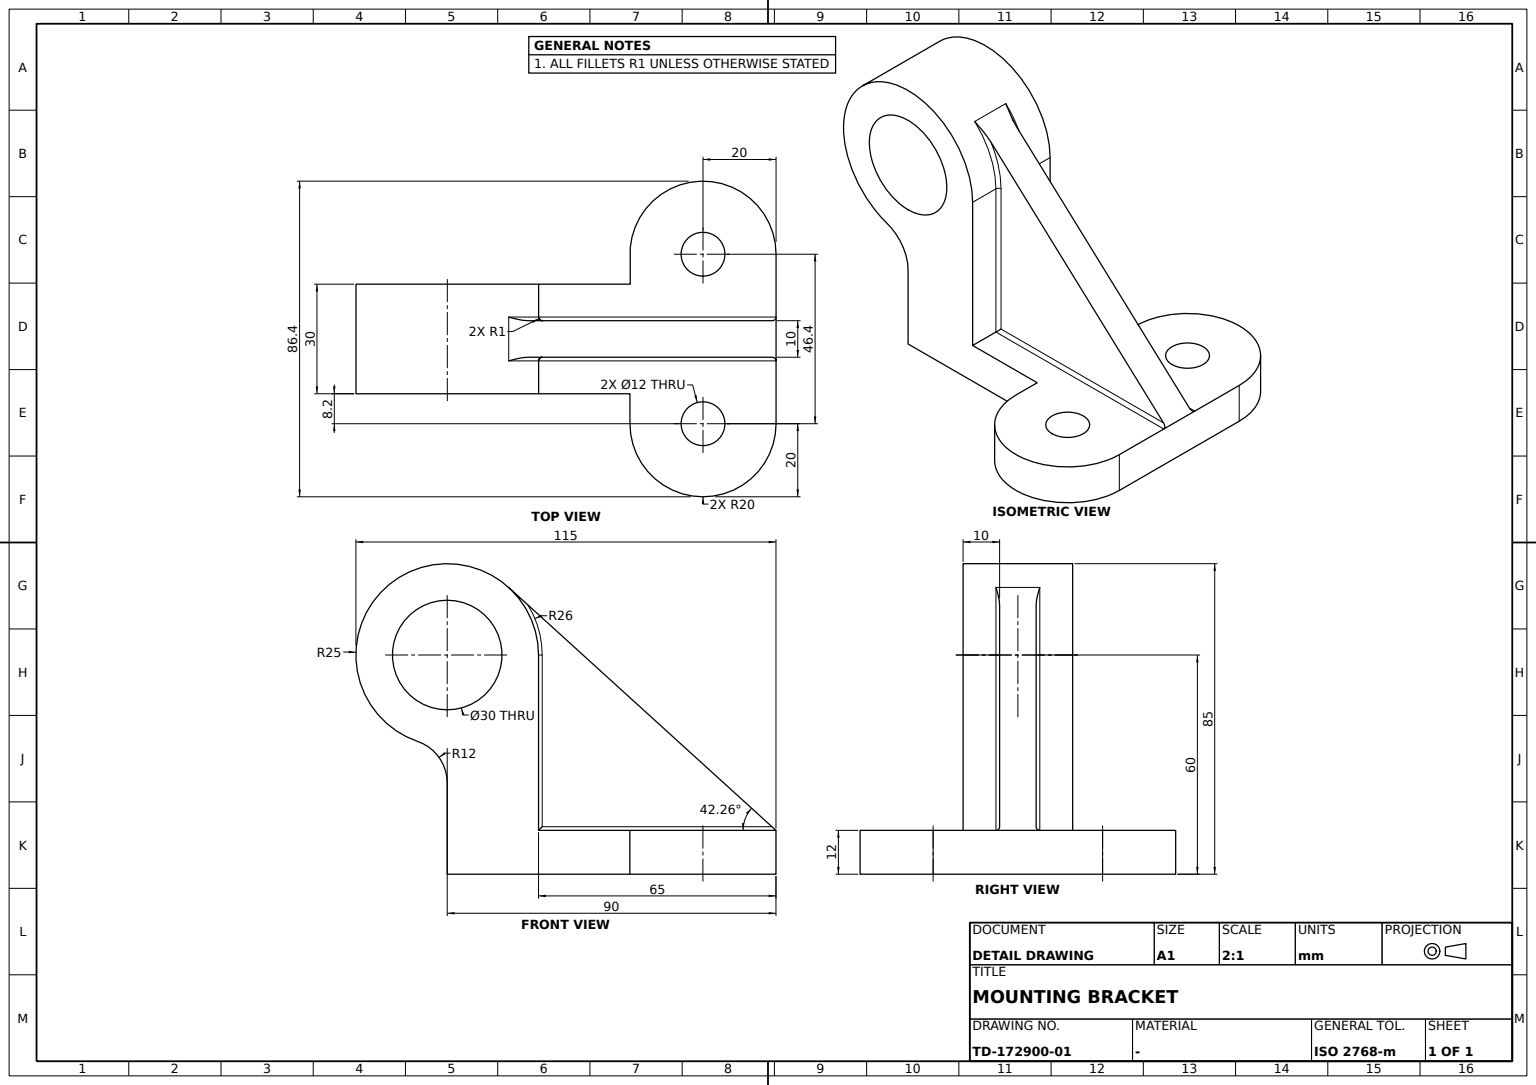
ISO-10303-21;
HEADER;
FILE_DESCRIPTION((''),'2;1');
FILE_NAME('','',(''),(''),'','','');
FILE_SCHEMA(('AUTOMOTIVE_DESIGN'));
ENDSEC;
DATA;
#1=APPLICATION_CONTEXT('');
#2=PRODUCT_CONTEXT('',#1,'mechanical');
#3=PRODUCT('','','',(#2));
#4=PRODUCT_DEFINITION_FORMATION('','',#3);
#5=PRODUCT_DEFINITION_CONTEXT('',#1,'design');
#6=PRODUCT_DEFINITION('','',#4,#5);
#7=PRODUCT_DEFINITION_SHAPE('','',#6);
#8=(LENGTH_UNIT()NAMED_UNIT(*)SI_UNIT(.MILLI.,.METRE.));
#9=(NAMED_UNIT(*)PLANE_ANGLE_UNIT()SI_UNIT($,.RADIAN.));
#10=(NAMED_UNIT(*)SI_UNIT($,.STERADIAN.)SOLID_ANGLE_UNIT());
#11=UNCERTAINTY_MEASURE_WITH_UNIT(LENGTH_MEASURE(0.005),#8,'distance_accuracy_value','');
#12=(GEOMETRIC_REPRESENTATION_CONTEXT(3)GLOBAL_UNCERTAINTY_ASSIGNED_CONTEXT((#11))GLOBAL_UNIT_ASSIGNED_CONTEXT((#8,#9,#10))REPRESENTATION_CONTEXT('',''));
#13=CARTESIAN_POINT('',(23.199566,90.,-60.));
#14=VERTEX_POINT('',#13);
#15=CARTESIAN_POINT('',(23.199566,90.,-48.));
#16=VERTEX_POINT('',#15);
#17=CARTESIAN_POINT('',(23.199566,90.,-54.));
#18=DIRECTION('',(0.,0.,1.));
#19=VECTOR('',#18,1000.);
#20=LINE('',#17,#19);
#21=EDGE_CURVE('',#14,#16,#20,.T.);
#22=ORIENTED_EDGE('',*,*,#21,.F.);
#23=CARTESIAN_POINT('',(-23.199566,90.,-60.));
#24=VERTEX_POINT('',#23);
#25=CARTESIAN_POINT('',(0.,90.,-60.));
#26=DIRECTION('',(1.,0.,0.));
#27=VECTOR('',#26,1000.);
#28=LINE('',#25,#27);
#29=EDGE_CURVE('',#24,#14,#28,.T.);
#30=ORIENTED_EDGE('',*,*,#29,.F.);
#31=CARTESIAN_POINT('',(-23.199566,90.,-48.));
#32=VERTEX_POINT('',#31);
#33=CARTESIAN_POINT('',(-23.199566,90.,-54.));
#34=LINE('',#33,#19);
#35=EDGE_CURVE('',#24,#32,#34,.T.);
#36=ORIENTED_EDGE('',*,*,#35,.T.);
#37=CARTESIAN_POINT('',(-6.,90.,-48.));
#38=VERTEX_POINT('',#37);
#39=CARTESIAN_POINT('',(0.,90.,-48.));
#40=LINE('',#39,#27);
#41=EDGE_CURVE('',#32,#38,#40,.T.);
#42=ORIENTED_EDGE('',*,*,#41,.T.);
#43=CARTESIAN_POINT('',(6.,90.,-48.));
#44=VERTEX_POINT('',#43);
#45=LINE('',#31,#27);
#46=EDGE_CURVE('',#38,#44,#45,.T.);
#47=ORIENTED_EDGE('',*,*,#46,.T.);
#48=EDGE_CURVE('',#44,#16,#40,.T.);
#49=ORIENTED_EDGE('',*,*,#48,.T.);
#50=EDGE_LOOP('',(#22,#30,#36,#42,#47,#49));
#51=FACE_BOUND('',#50,.T.);
#52=DIRECTION('',(0.,-1.,0.));
#53=AXIS2_PLACEMENT_3D('',#23,#52,#26);
#54=PLANE('',#53);
#55=ADVANCED_FACE('',(#51),#54,.F.);
#56=CARTESIAN_POINT('',(-15.,0.,-15.));
#57=VERTEX_POINT('',#56);
#58=CARTESIAN_POINT('',(-15.,0.,0.));
#59=DIRECTION('',(0.,0.,-1.));
#60=AXIS2_PLACEMENT_3D('',#58,#26,#59);
#61=CIRCLE('',#60,15.);
#62=EDGE_CURVE('',#57,#57,#61,.T.);
#63=ORIENTED_EDGE('',*,*,#62,.F.);
#64=EDGE_LOOP('',(#63));
#65=FACE_BOUND('',#64,.T.);
#66=CARTESIAN_POINT('',(15.,0.,-15.));
#67=VERTEX_POINT('',#66);
#68=CARTESIAN_POINT('',(15.,0.,0.));
#69=AXIS2_PLACEMENT_3D('',#68,#26,#59);
#70=CIRCLE('',#69,15.);
#71=EDGE_CURVE('',#67,#67,#70,.T.);
#72=ORIENTED_EDGE('',*,*,#71,.T.);
#73=EDGE_LOOP('',(#72));
#74=FACE_BOUND('',#73,.T.);
#75=CARTESIAN_POINT('',(0.,0.,0.));
#76=DIRECTION('',(0.,1.,0.));
#77=AXIS2_PLACEMENT_3D('',#75,#26,#76);
#78=CYLINDRICAL_SURFACE('',#77,15.);
#79=ADVANCED_FACE('',(#65,#74),#78,.F.);
#80=CARTESIAN_POINT('',(29.199566,70.,-60.));
#81=VERTEX_POINT('',#80);
#82=CARTESIAN_POINT('',(23.199566,70.,-60.));
#83=AXIS2_PLACEMENT_3D('',#82,#18,#26);
#84=CIRCLE('',#83,6.);
#85=EDGE_CURVE('',#81,#81,#84,.T.);
#86=ORIENTED_EDGE('',*,*,#85,.T.);
#87=EDGE_LOOP('',(#86));
#88=FACE_BOUND('',#87,.T.);
#89=CARTESIAN_POINT('',(23.199566,50.,-60.));
#90=VERTEX_POINT('',#89);
#91=CIRCLE('',#83,20.);
#92=EDGE_CURVE('',#90,#14,#91,.T.);
#93=ORIENTED_EDGE('',*,*,#92,.F.);
#94=CARTESIAN_POINT('',(15.,50.,-60.));
#95=VERTEX_POINT('',#94);
#96=CARTESIAN_POINT('',(0.,50.,-60.));
#97=DIRECTION('',(-1.,0.,0.));
#98=VECTOR('',#97,1000.);
#99=LINE('',#96,#98);
#100=EDGE_CURVE('',#90,#95,#99,.T.);
#101=ORIENTED_EDGE('',*,*,#100,.T.);
#102=CARTESIAN_POINT('',(15.,0.,-60.));
#103=VERTEX_POINT('',#102);
#104=VECTOR('',#52,1000.);
#105=LINE('',#102,#104);
#106=EDGE_CURVE('',#95,#103,#105,.T.);
#107=ORIENTED_EDGE('',*,*,#106,.T.);
#108=CARTESIAN_POINT('',(-15.,0.,-60.));
#109=VERTEX_POINT('',#108);
#110=CARTESIAN_POINT('',(0.,0.,-60.));
#111=LINE('',#110,#27);
#112=EDGE_CURVE('',#109,#103,#111,.T.);
#113=ORIENTED_EDGE('',*,*,#112,.F.);
#114=CARTESIAN_POINT('',(-15.,50.081204,-60.));
#115=VERTEX_POINT('',#114);
#116=LINE('',#108,#104);
#117=EDGE_CURVE('',#115,#109,#116,.T.);
#118=ORIENTED_EDGE('',*,*,#117,.F.);
#119=CARTESIAN_POINT('',(-25.,50.081204,-60.));
#120=VERTEX_POINT('',#119);
#121=CARTESIAN_POINT('',(0.,50.081204,-60.));
#122=LINE('',#121,#27);
#123=EDGE_CURVE('',#120,#115,#122,.T.);
#124=ORIENTED_EDGE('',*,*,#123,.F.);
#125=CARTESIAN_POINT('',(-23.199566,70.,-60.));
#126=AXIS2_PLACEMENT_3D('',#125,#18,#26);
#127=CIRCLE('',#126,20.);
#128=EDGE_CURVE('',#24,#120,#127,.T.);
#129=ORIENTED_EDGE('',*,*,#128,.F.);
#130=ORIENTED_EDGE('',*,*,#29,.T.);
#131=EDGE_LOOP('',(#93,#101,#107,#113,#118,#124,#129,#130));
#132=FACE_BOUND('',#131,.T.);
#133=CARTESIAN_POINT('',(-17.199566,70.,-60.));
#134=VERTEX_POINT('',#133);
#135=CIRCLE('',#126,6.);
#136=EDGE_CURVE('',#134,#134,#135,.T.);
#137=ORIENTED_EDGE('',*,*,#136,.T.);
#138=EDGE_LOOP('',(#137));
#139=FACE_BOUND('',#138,.T.);
#140=CARTESIAN_POINT('',(0.,25.,-60.));
#141=AXIS2_PLACEMENT_3D('',#140,#18,#52);
#142=PLANE('',#141);
#143=ADVANCED_FACE('',(#88,#132,#139),#142,.F.);
#144=ORIENTED_EDGE('',*,*,#85,.F.);
#145=EDGE_LOOP('',(#144));
#146=FACE_BOUND('',#145,.T.);
#147=CARTESIAN_POINT('',(29.199566,70.,-48.));
#148=VERTEX_POINT('',#147);
#149=CARTESIAN_POINT('',(23.199566,70.,-48.));
#150=AXIS2_PLACEMENT_3D('',#149,#18,#26);
#151=CIRCLE('',#150,6.);
#152=EDGE_CURVE('',#148,#148,#151,.T.);
#153=ORIENTED_EDGE('',*,*,#152,.T.);
#154=EDGE_LOOP('',(#153));
#155=FACE_BOUND('',#154,.T.);
#156=CARTESIAN_POINT('',(23.199566,70.,-54.));
#157=AXIS2_PLACEMENT_3D('',#156,#18,#76);
#158=CYLINDRICAL_SURFACE('',#157,6.);
#159=ADVANCED_FACE('',(#146,#155),#158,.F.);
#160=CARTESIAN_POINT('',(15.,-8.108108,-23.648649));
#161=VERTEX_POINT('',#160);
#162=CARTESIAN_POINT('',(-15.,-8.108108,-23.648649));
#163=VERTEX_POINT('',#162);
#164=CARTESIAN_POINT('',(0.,-8.108108,-23.648649));
#165=LINE('',#164,#27);
#166=EDGE_CURVE('',#161,#163,#165,.F.);
#167=ORIENTED_EDGE('',*,*,#166,.T.);
#168=CARTESIAN_POINT('',(-15.,0.,-35.));
#169=VERTEX_POINT('',#168);
#170=CARTESIAN_POINT('',(-15.,-12.,-35.));
#171=AXIS2_PLACEMENT_3D('',#170,#26,#59);
#172=CIRCLE('',#171,12.);
#173=EDGE_CURVE('',#169,#163,#172,.T.);
#174=ORIENTED_EDGE('',*,*,#173,.F.);
#175=CARTESIAN_POINT('',(15.,0.,-35.));
#176=VERTEX_POINT('',#175);
#177=CARTESIAN_POINT('',(0.,0.,-35.));
#178=LINE('',#177,#98);
#179=EDGE_CURVE('',#176,#169,#178,.T.);
#180=ORIENTED_EDGE('',*,*,#179,.F.);
#181=CARTESIAN_POINT('',(15.,-12.,-35.));
#182=AXIS2_PLACEMENT_3D('',#181,#26,#59);
#183=CIRCLE('',#182,12.);
#184=EDGE_CURVE('',#176,#161,#183,.T.);
#185=ORIENTED_EDGE('',*,*,#184,.T.);
#186=EDGE_LOOP('',(#167,#174,#180,#185));
#187=FACE_BOUND('',#186,.T.);
#188=CARTESIAN_POINT('',(0.,-12.,-35.));
#189=AXIS2_PLACEMENT_3D('',#188,#97,#76);
#190=CYLINDRICAL_SURFACE('',#189,12.);
#191=ADVANCED_FACE('',(#187),#190,.F.);
#192=CARTESIAN_POINT('',(-25.,50.081204,-48.));
#193=VERTEX_POINT('',#192);
#194=CARTESIAN_POINT('',(-23.199566,70.,-48.));
#195=AXIS2_PLACEMENT_3D('',#194,#18,#26);
#196=CIRCLE('',#195,20.);
#197=EDGE_CURVE('',#32,#193,#196,.T.);
#198=ORIENTED_EDGE('',*,*,#197,.F.);
#199=ORIENTED_EDGE('',*,*,#35,.F.);
#200=ORIENTED_EDGE('',*,*,#128,.T.);
#201=LINE('',#119,#19);
#202=EDGE_CURVE('',#120,#193,#201,.T.);
#203=ORIENTED_EDGE('',*,*,#202,.T.);
#204=EDGE_LOOP('',(#198,#199,#200,#203));
#205=FACE_BOUND('',#204,.T.);
#206=CARTESIAN_POINT('',(-23.199566,70.,-54.));
#207=AXIS2_PLACEMENT_3D('',#206,#18,#76);
#208=CYLINDRICAL_SURFACE('',#207,20.);
#209=ADVANCED_FACE('',(#205),#208,.T.);
#210=CARTESIAN_POINT('',(-6.,25.,0.));
#211=VERTEX_POINT('',#210);
#212=CARTESIAN_POINT('',(-6.,25.,-48.));
#213=VERTEX_POINT('',#212);
#214=CARTESIAN_POINT('',(-6.,25.,-14.748757));
#215=VECTOR('',#59,1000.);
#216=LINE('',#214,#215);
#217=EDGE_CURVE('',#211,#213,#216,.T.);
#218=ORIENTED_EDGE('',*,*,#217,.F.);
#219=CARTESIAN_POINT('',(-5.,26.,0.));
#220=VERTEX_POINT('',#219);
#221=CARTESIAN_POINT('',(-6.,26.,0.));
#222=AXIS2_PLACEMENT_3D('',#221,#59,#97);
#223=CIRCLE('',#222,1.);
#224=EDGE_CURVE('',#220,#211,#223,.T.);
#225=ORIENTED_EDGE('',*,*,#224,.F.);
#226=CARTESIAN_POINT('',(-5.,26.,-47.));
#227=VERTEX_POINT('',#226);
#228=CARTESIAN_POINT('',(-5.,26.,-14.748757));
#229=LINE('',#228,#215);
#230=EDGE_CURVE('',#220,#227,#229,.T.);
#231=ORIENTED_EDGE('',*,*,#230,.T.);
#232=CARTESIAN_POINT('',(-6.,26.,-47.));
#233=DIRECTION('',(0.,0.707106781,-0.707106781));
#234=DIRECTION('',(0.,-0.707106781,-0.707106781));
#235=AXIS2_PLACEMENT_3D('',#232,#233,#234);
#236=ELLIPSE('',#235,1.414214,1.);
#237=EDGE_CURVE('',#227,#213,#236,.T.);
#238=ORIENTED_EDGE('',*,*,#237,.T.);
#239=EDGE_LOOP('',(#218,#225,#231,#238));
#240=FACE_BOUND('',#239,.T.);
#241=CARTESIAN_POINT('',(-6.,26.,-14.748757));
#242=AXIS2_PLACEMENT_3D('',#241,#59,#26);
#243=CYLINDRICAL_SURFACE('',#242,1.);
#244=ADVANCED_FACE('',(#240),#243,.F.);
#245=CARTESIAN_POINT('',(-15.,50.081204,-48.));
#246=VERTEX_POINT('',#245);
#247=LINE('',#114,#19);
#248=EDGE_CURVE('',#115,#246,#247,.T.);
#249=ORIENTED_EDGE('',*,*,#248,.T.);
#250=CARTESIAN_POINT('',(0.,50.081204,-48.));
#251=LINE('',#250,#27);
#252=EDGE_CURVE('',#193,#246,#251,.T.);
#253=ORIENTED_EDGE('',*,*,#252,.F.);
#254=ORIENTED_EDGE('',*,*,#202,.F.);
#255=ORIENTED_EDGE('',*,*,#123,.T.);
#256=EDGE_LOOP('',(#249,#253,#254,#255));
#257=FACE_BOUND('',#256,.T.);
#258=AXIS2_PLACEMENT_3D('',#119,#52,#26);
#259=PLANE('',#258);
#260=ADVANCED_FACE('',(#257),#259,.T.);
#261=CARTESIAN_POINT('',(5.,26.,0.));
#262=VERTEX_POINT('',#261);
#263=CARTESIAN_POINT('',(5.,22.097804,13.699893));
#264=VERTEX_POINT('',#263);
#265=CARTESIAN_POINT('',(5.,0.,0.));
#266=AXIS2_PLACEMENT_3D('',#265,#26,#59);
#267=CIRCLE('',#266,26.);
#268=EDGE_CURVE('',#262,#264,#267,.T.);
#269=ORIENTED_EDGE('',*,*,#268,.T.);
#270=CARTESIAN_POINT('',(6.,16.812437,18.502486));
#271=VERTEX_POINT('',#270);
#272=CARTESIAN_POINT('',(5.,20.312619,15.322016));
#273=CARTESIAN_POINT('',(5.527816,18.559761,16.914765));
#274=B_SPLINE_CURVE_WITH_KNOTS('',3,(#263,#272,#273,#270),.UNSPECIFIED.,.F.,.F.,(4,4),(0.,0.00722306),.UNSPECIFIED.);
#275=EDGE_CURVE('',#264,#271,#274,.T.);
#276=ORIENTED_EDGE('',*,*,#275,.T.);
#277=CARTESIAN_POINT('',(6.,25.,0.));
#278=VERTEX_POINT('',#277);
#279=CARTESIAN_POINT('',(6.,0.,0.));
#280=AXIS2_PLACEMENT_3D('',#279,#26,#59);
#281=CIRCLE('',#280,25.);
#282=EDGE_CURVE('',#278,#271,#281,.T.);
#283=ORIENTED_EDGE('',*,*,#282,.F.);
#284=CARTESIAN_POINT('',(6.,26.,0.));
#285=AXIS2_PLACEMENT_3D('',#284,#18,#26);
#286=CIRCLE('',#285,1.);
#287=EDGE_CURVE('',#278,#262,#286,.F.);
#288=ORIENTED_EDGE('',*,*,#287,.T.);
#289=EDGE_LOOP('',(#269,#276,#283,#288));
#290=FACE_BOUND('',#289,.T.);
#291=DIRECTION('',(0.,0.758530448,-0.651637599));
#292=AXIS2_PLACEMENT_3D('',#279,#26,#291);
#293=TOROIDAL_SURFACE('',#292,26.,1.);
#294=ADVANCED_FACE('',(#290),#293,.F.);
#295=ORIENTED_EDGE('',*,*,#237,.F.);
#296=CARTESIAN_POINT('',(-5.,88.899476,-47.));
#297=VERTEX_POINT('',#296);
#298=CARTESIAN_POINT('',(-5.,53.406218,-47.));
#299=VECTOR('',#76,1000.);
#300=LINE('',#298,#299);
#301=EDGE_CURVE('',#227,#297,#300,.T.);
#302=ORIENTED_EDGE('',*,*,#301,.T.);
#303=CARTESIAN_POINT('',(-6.,88.899476,-47.));
#304=DIRECTION('',(0.,-0.672497469,-0.740099422));
#305=DIRECTION('',(0.,0.740099422,-0.672497469));
#306=AXIS2_PLACEMENT_3D('',#303,#304,#305);
#307=ELLIPSE('',#306,1.486994,1.);
#308=EDGE_CURVE('',#297,#38,#307,.F.);
#309=ORIENTED_EDGE('',*,*,#308,.T.);
#310=CARTESIAN_POINT('',(-6.,53.406218,-48.));
#311=LINE('',#310,#299);
#312=EDGE_CURVE('',#213,#38,#311,.T.);
#313=ORIENTED_EDGE('',*,*,#312,.F.);
#314=EDGE_LOOP('',(#295,#302,#309,#313));
#315=FACE_BOUND('',#314,.T.);
#316=CARTESIAN_POINT('',(-6.,53.406218,-47.));
#317=AXIS2_PLACEMENT_3D('',#316,#76,#26);
#318=CYLINDRICAL_SURFACE('',#317,1.);
#319=ADVANCED_FACE('',(#315),#318,.F.);
#320=CARTESIAN_POINT('',(-15.,25.,0.));
#321=VERTEX_POINT('',#320);
#322=CARTESIAN_POINT('',(0.,25.,0.));
#323=LINE('',#322,#27);
#324=EDGE_CURVE('',#321,#211,#323,.T.);
#325=ORIENTED_EDGE('',*,*,#324,.T.);
#326=ORIENTED_EDGE('',*,*,#217,.T.);
#327=CARTESIAN_POINT('',(-15.,25.,-48.));
#328=VERTEX_POINT('',#327);
#329=CARTESIAN_POINT('',(0.,25.,-48.));
#330=LINE('',#329,#27);
#331=EDGE_CURVE('',#328,#213,#330,.T.);
#332=ORIENTED_EDGE('',*,*,#331,.F.);
#333=LINE('',#320,#215);
#334=EDGE_CURVE('',#321,#328,#333,.T.);
#335=ORIENTED_EDGE('',*,*,#334,.F.);
#336=EDGE_LOOP('',(#325,#326,#332,#335));
#337=FACE_BOUND('',#336,.T.);
#338=AXIS2_PLACEMENT_3D('',#322,#52,#59);
#339=PLANE('',#338);
#340=ADVANCED_FACE('',(#337),#339,.F.);
#341=CARTESIAN_POINT('',(-5.,22.097804,13.699893));
#342=VERTEX_POINT('',#341);
#343=CARTESIAN_POINT('',(-5.,16.812437,18.502486));
#344=VECTOR('',#305,1000.);
#345=LINE('',#343,#344);
#346=EDGE_CURVE('',#342,#297,#345,.T.);
#347=ORIENTED_EDGE('',*,*,#346,.T.);
#348=ORIENTED_EDGE('',*,*,#301,.F.);
#349=ORIENTED_EDGE('',*,*,#230,.F.);
#350=CARTESIAN_POINT('',(-5.,0.,0.));
#351=AXIS2_PLACEMENT_3D('',#350,#26,#59);
#352=CIRCLE('',#351,26.);
#353=EDGE_CURVE('',#220,#342,#352,.T.);
#354=ORIENTED_EDGE('',*,*,#353,.T.);
#355=EDGE_LOOP('',(#347,#348,#349,#354));
#356=FACE_BOUND('',#355,.T.);
#357=AXIS2_PLACEMENT_3D('',#350,#26,#76);
#358=PLANE('',#357);
#359=ADVANCED_FACE('',(#356),#358,.F.);
#360=ORIENTED_EDGE('',*,*,#152,.F.);
#361=EDGE_LOOP('',(#360));
#362=FACE_BOUND('',#361,.T.);
#363=CARTESIAN_POINT('',(6.,25.,-48.));
#364=VERTEX_POINT('',#363);
#365=CARTESIAN_POINT('',(15.,25.,-48.));
#366=VERTEX_POINT('',#365);
#367=EDGE_CURVE('',#364,#366,#330,.T.);
#368=ORIENTED_EDGE('',*,*,#367,.T.);
#369=CARTESIAN_POINT('',(15.,50.,-48.));
#370=VERTEX_POINT('',#369);
#371=CARTESIAN_POINT('',(15.,0.,-48.));
#372=LINE('',#371,#299);
#373=EDGE_CURVE('',#366,#370,#372,.T.);
#374=ORIENTED_EDGE('',*,*,#373,.T.);
#375=CARTESIAN_POINT('',(23.199566,50.,-48.));
#376=VERTEX_POINT('',#375);
#377=CARTESIAN_POINT('',(0.,50.,-48.));
#378=LINE('',#377,#98);
#379=EDGE_CURVE('',#376,#370,#378,.T.);
#380=ORIENTED_EDGE('',*,*,#379,.F.);
#381=CIRCLE('',#150,20.);
#382=EDGE_CURVE('',#376,#16,#381,.T.);
#383=ORIENTED_EDGE('',*,*,#382,.T.);
#384=ORIENTED_EDGE('',*,*,#48,.F.);
#385=CARTESIAN_POINT('',(6.,53.406218,-48.));
#386=LINE('',#385,#299);
#387=EDGE_CURVE('',#364,#44,#386,.T.);
#388=ORIENTED_EDGE('',*,*,#387,.F.);
#389=EDGE_LOOP('',(#368,#374,#380,#383,#384,#388));
#390=FACE_BOUND('',#389,.T.);
#391=CARTESIAN_POINT('',(0.,0.,-48.));
#392=AXIS2_PLACEMENT_3D('',#391,#18,#76);
#393=PLANE('',#392);
#394=ADVANCED_FACE('',(#362,#390),#393,.T.);
#395=CARTESIAN_POINT('',(15.,25.,0.));
#396=VERTEX_POINT('',#395);
#397=CIRCLE('',#69,25.);
#398=EDGE_CURVE('',#396,#161,#397,.T.);
#399=ORIENTED_EDGE('',*,*,#398,.F.);
#400=EDGE_CURVE('',#278,#396,#323,.T.);
#401=ORIENTED_EDGE('',*,*,#400,.F.);
#402=ORIENTED_EDGE('',*,*,#282,.T.);
#403=CARTESIAN_POINT('',(-6.,16.812437,18.502486));
#404=VERTEX_POINT('',#403);
#405=CARTESIAN_POINT('',(0.,16.812437,18.502486));
#406=LINE('',#405,#27);
#407=EDGE_CURVE('',#404,#271,#406,.T.);
#408=ORIENTED_EDGE('',*,*,#407,.F.);
#409=CARTESIAN_POINT('',(-6.,0.,0.));
#410=AXIS2_PLACEMENT_3D('',#409,#26,#59);
#411=CIRCLE('',#410,25.);
#412=EDGE_CURVE('',#211,#404,#411,.T.);
#413=ORIENTED_EDGE('',*,*,#412,.F.);
#414=ORIENTED_EDGE('',*,*,#324,.F.);
#415=CIRCLE('',#60,25.);
#416=EDGE_CURVE('',#321,#163,#415,.T.);
#417=ORIENTED_EDGE('',*,*,#416,.T.);
#418=ORIENTED_EDGE('',*,*,#166,.F.);
#419=EDGE_LOOP('',(#399,#401,#402,#408,#413,#414,#417,#418));
#420=FACE_BOUND('',#419,.T.);
#421=CYLINDRICAL_SURFACE('',#77,25.);
#422=ADVANCED_FACE('',(#420),#421,.T.);
#423=CARTESIAN_POINT('',(5.,26.,-47.));
#424=VERTEX_POINT('',#423);
#425=CARTESIAN_POINT('',(5.,88.899476,-47.));
#426=VERTEX_POINT('',#425);
#427=CARTESIAN_POINT('',(5.,53.406218,-47.));
#428=LINE('',#427,#299);
#429=EDGE_CURVE('',#424,#426,#428,.T.);
#430=ORIENTED_EDGE('',*,*,#429,.F.);
#431=CARTESIAN_POINT('',(6.,26.,-47.));
#432=DIRECTION('',(0.,0.707106781,0.707106781));
#433=AXIS2_PLACEMENT_3D('',#431,#233,#432);
#434=ELLIPSE('',#433,1.414214,1.);
#435=EDGE_CURVE('',#424,#364,#434,.F.);
#436=ORIENTED_EDGE('',*,*,#435,.T.);
#437=ORIENTED_EDGE('',*,*,#387,.T.);
#438=CARTESIAN_POINT('',(6.,88.899476,-47.));
#439=AXIS2_PLACEMENT_3D('',#438,#304,#305);
#440=ELLIPSE('',#439,1.486994,1.);
#441=EDGE_CURVE('',#426,#44,#440,.T.);
#442=ORIENTED_EDGE('',*,*,#441,.F.);
#443=EDGE_LOOP('',(#430,#436,#437,#442));
#444=FACE_BOUND('',#443,.T.);
#445=CARTESIAN_POINT('',(6.,53.406218,-47.));
#446=AXIS2_PLACEMENT_3D('',#445,#76,#59);
#447=CYLINDRICAL_SURFACE('',#446,1.);
#448=ADVANCED_FACE('',(#444),#447,.F.);
#449=CARTESIAN_POINT('',(-17.199566,70.,-48.));
#450=VERTEX_POINT('',#449);
#451=CIRCLE('',#195,6.);
#452=EDGE_CURVE('',#450,#450,#451,.T.);
#453=ORIENTED_EDGE('',*,*,#452,.F.);
#454=EDGE_LOOP('',(#453));
#455=FACE_BOUND('',#454,.T.);
#456=ORIENTED_EDGE('',*,*,#41,.F.);
#457=ORIENTED_EDGE('',*,*,#197,.T.);
#458=ORIENTED_EDGE('',*,*,#252,.T.);
#459=CARTESIAN_POINT('',(-15.,0.,-48.));
#460=LINE('',#459,#299);
#461=EDGE_CURVE('',#328,#246,#460,.T.);
#462=ORIENTED_EDGE('',*,*,#461,.F.);
#463=ORIENTED_EDGE('',*,*,#331,.T.);
#464=ORIENTED_EDGE('',*,*,#312,.T.);
#465=EDGE_LOOP('',(#456,#457,#458,#462,#463,#464));
#466=FACE_BOUND('',#465,.T.);
#467=ADVANCED_FACE('',(#455,#466),#393,.T.);
#468=LINE('',#68,#19);
#469=EDGE_CURVE('',#103,#176,#468,.T.);
#470=ORIENTED_EDGE('',*,*,#469,.F.);
#471=ORIENTED_EDGE('',*,*,#106,.F.);
#472=CARTESIAN_POINT('',(15.,50.,0.));
#473=LINE('',#472,#19);
#474=EDGE_CURVE('',#95,#370,#473,.T.);
#475=ORIENTED_EDGE('',*,*,#474,.T.);
#476=ORIENTED_EDGE('',*,*,#373,.F.);
#477=LINE('',#395,#215);
#478=EDGE_CURVE('',#396,#366,#477,.T.);
#479=ORIENTED_EDGE('',*,*,#478,.F.);
#480=ORIENTED_EDGE('',*,*,#398,.T.);
#481=ORIENTED_EDGE('',*,*,#184,.F.);
#482=EDGE_LOOP('',(#470,#471,#475,#476,#479,#480,#481));
#483=FACE_BOUND('',#482,.T.);
#484=ORIENTED_EDGE('',*,*,#71,.F.);
#485=EDGE_LOOP('',(#484));
#486=FACE_BOUND('',#485,.T.);
#487=AXIS2_PLACEMENT_3D('',#68,#26,#76);
#488=PLANE('',#487);
#489=ADVANCED_FACE('',(#483,#486),#488,.T.);
#490=ORIENTED_EDGE('',*,*,#62,.T.);
#491=EDGE_LOOP('',(#490));
#492=FACE_BOUND('',#491,.T.);
#493=ORIENTED_EDGE('',*,*,#416,.F.);
#494=ORIENTED_EDGE('',*,*,#334,.T.);
#495=ORIENTED_EDGE('',*,*,#461,.T.);
#496=ORIENTED_EDGE('',*,*,#248,.F.);
#497=ORIENTED_EDGE('',*,*,#117,.T.);
#498=LINE('',#58,#19);
#499=EDGE_CURVE('',#109,#169,#498,.T.);
#500=ORIENTED_EDGE('',*,*,#499,.T.);
#501=ORIENTED_EDGE('',*,*,#173,.T.);
#502=EDGE_LOOP('',(#493,#494,#495,#496,#497,#500,#501));
#503=FACE_BOUND('',#502,.T.);
#504=AXIS2_PLACEMENT_3D('',#58,#26,#76);
#505=PLANE('',#504);
#506=ADVANCED_FACE('',(#492,#503),#505,.F.);
#507=CARTESIAN_POINT('',(6.,25.,-14.748757));
#508=LINE('',#507,#19);
#509=EDGE_CURVE('',#364,#278,#508,.T.);
#510=ORIENTED_EDGE('',*,*,#509,.F.);
#511=ORIENTED_EDGE('',*,*,#435,.F.);
#512=CARTESIAN_POINT('',(5.,26.,-14.748757));
#513=LINE('',#512,#19);
#514=EDGE_CURVE('',#424,#262,#513,.T.);
#515=ORIENTED_EDGE('',*,*,#514,.T.);
#516=ORIENTED_EDGE('',*,*,#287,.F.);
#517=EDGE_LOOP('',(#510,#511,#515,#516));
#518=FACE_BOUND('',#517,.T.);
#519=CARTESIAN_POINT('',(6.,26.,-14.748757));
#520=AXIS2_PLACEMENT_3D('',#519,#18,#52);
#521=CYLINDRICAL_SURFACE('',#520,1.);
#522=ADVANCED_FACE('',(#518),#521,.F.);
#523=ORIENTED_EDGE('',*,*,#382,.F.);
#524=CARTESIAN_POINT('',(23.199566,50.,-54.));
#525=LINE('',#524,#19);
#526=EDGE_CURVE('',#90,#376,#525,.T.);
#527=ORIENTED_EDGE('',*,*,#526,.F.);
#528=ORIENTED_EDGE('',*,*,#92,.T.);
#529=ORIENTED_EDGE('',*,*,#21,.T.);
#530=EDGE_LOOP('',(#523,#527,#528,#529));
#531=FACE_BOUND('',#530,.T.);
#532=CYLINDRICAL_SURFACE('',#157,20.);
#533=ADVANCED_FACE('',(#531),#532,.T.);
#534=ORIENTED_EDGE('',*,*,#478,.T.);
#535=ORIENTED_EDGE('',*,*,#367,.F.);
#536=ORIENTED_EDGE('',*,*,#509,.T.);
#537=ORIENTED_EDGE('',*,*,#400,.T.);
#538=EDGE_LOOP('',(#534,#535,#536,#537));
#539=FACE_BOUND('',#538,.T.);
#540=ADVANCED_FACE('',(#539),#339,.F.);
#541=ORIENTED_EDGE('',*,*,#100,.F.);
#542=ORIENTED_EDGE('',*,*,#526,.T.);
#543=ORIENTED_EDGE('',*,*,#379,.T.);
#544=ORIENTED_EDGE('',*,*,#474,.F.);
#545=EDGE_LOOP('',(#541,#542,#543,#544));
#546=FACE_BOUND('',#545,.T.);
#547=AXIS2_PLACEMENT_3D('',#89,#76,#97);
#548=PLANE('',#547);
#549=ADVANCED_FACE('',(#546),#548,.F.);
#550=ORIENTED_EDGE('',*,*,#514,.F.);
#551=ORIENTED_EDGE('',*,*,#429,.T.);
#552=CARTESIAN_POINT('',(5.,16.812437,18.502486));
#553=LINE('',#552,#344);
#554=EDGE_CURVE('',#264,#426,#553,.T.);
#555=ORIENTED_EDGE('',*,*,#554,.F.);
#556=ORIENTED_EDGE('',*,*,#268,.F.);
#557=EDGE_LOOP('',(#550,#551,#555,#556));
#558=FACE_BOUND('',#557,.T.);
#559=AXIS2_PLACEMENT_3D('',#265,#26,#76);
#560=PLANE('',#559);
#561=ADVANCED_FACE('',(#558),#560,.T.);
#562=ORIENTED_EDGE('',*,*,#224,.T.);
#563=ORIENTED_EDGE('',*,*,#412,.T.);
#564=CARTESIAN_POINT('',(-5.,20.312619,15.322016));
#565=CARTESIAN_POINT('',(-5.527816,18.559761,16.914765));
#566=B_SPLINE_CURVE_WITH_KNOTS('',3,(#341,#564,#565,#403),.UNSPECIFIED.,.F.,.F.,(4,4),(0.,0.00722306),.UNSPECIFIED.);
#567=EDGE_CURVE('',#342,#404,#566,.T.);
#568=ORIENTED_EDGE('',*,*,#567,.F.);
#569=ORIENTED_EDGE('',*,*,#353,.F.);
#570=EDGE_LOOP('',(#562,#563,#568,#569));
#571=FACE_BOUND('',#570,.T.);
#572=AXIS2_PLACEMENT_3D('',#409,#26,#291);
#573=TOROIDAL_SURFACE('',#572,26.,1.);
#574=ADVANCED_FACE('',(#571),#573,.F.);
#575=ORIENTED_EDGE('',*,*,#179,.T.);
#576=ORIENTED_EDGE('',*,*,#499,.F.);
#577=ORIENTED_EDGE('',*,*,#112,.T.);
#578=ORIENTED_EDGE('',*,*,#469,.T.);
#579=EDGE_LOOP('',(#575,#576,#577,#578));
#580=FACE_BOUND('',#579,.T.);
#581=AXIS2_PLACEMENT_3D('',#110,#76,#18);
#582=PLANE('',#581);
#583=ADVANCED_FACE('',(#580),#582,.F.);
#584=ORIENTED_EDGE('',*,*,#441,.T.);
#585=ORIENTED_EDGE('',*,*,#46,.F.);
#586=ORIENTED_EDGE('',*,*,#308,.F.);
#587=ORIENTED_EDGE('',*,*,#346,.F.);
#588=ORIENTED_EDGE('',*,*,#567,.T.);
#589=ORIENTED_EDGE('',*,*,#407,.T.);
#590=ORIENTED_EDGE('',*,*,#275,.F.);
#591=ORIENTED_EDGE('',*,*,#554,.T.);
#592=EDGE_LOOP('',(#584,#585,#586,#587,#588,#589,#590,#591));
#593=FACE_BOUND('',#592,.T.);
#594=AXIS2_PLACEMENT_3D('',#405,#304,#305);
#595=PLANE('',#594);
#596=ADVANCED_FACE('',(#593),#595,.F.);
#597=ORIENTED_EDGE('',*,*,#452,.T.);
#598=EDGE_LOOP('',(#597));
#599=FACE_BOUND('',#598,.T.);
#600=ORIENTED_EDGE('',*,*,#136,.F.);
#601=EDGE_LOOP('',(#600));
#602=FACE_BOUND('',#601,.T.);
#603=CYLINDRICAL_SURFACE('',#207,6.);
#604=ADVANCED_FACE('',(#599,#602),#603,.F.);
#605=CLOSED_SHELL('',(#55,#79,#143,#159,#191,#209,#244,#260,#294,#319,#340,#359,#394,#422,#448,#467,#489,#506,#522,#533,#540,#549,#561,#574,#583,#596,#604));
#606=MANIFOLD_SOLID_BREP('',#605);
#607=ADVANCED_BREP_SHAPE_REPRESENTATION('',(#606),#12);
#608=SHAPE_DEFINITION_REPRESENTATION(#7,#607);
ENDSEC;
END-ISO-10303-21;
